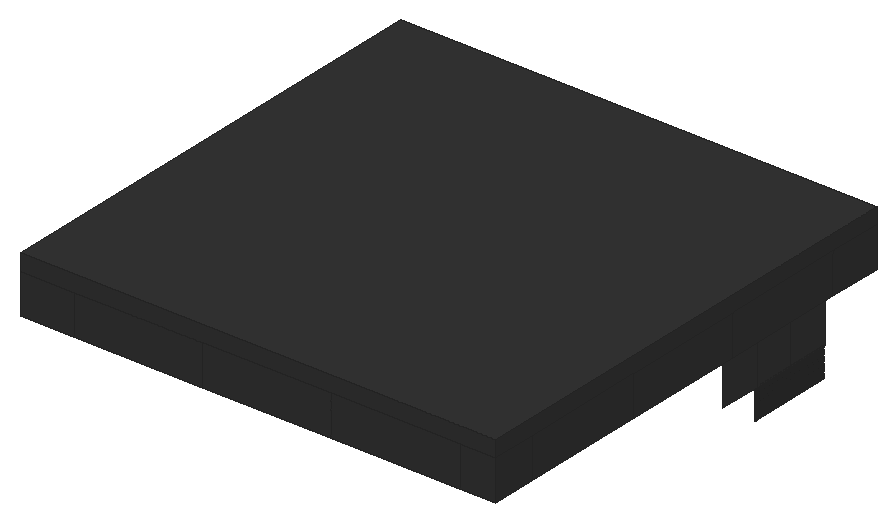
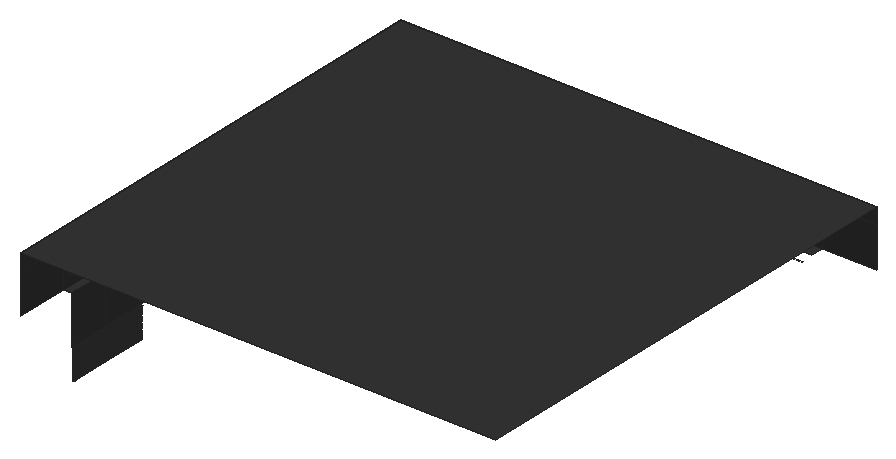
# SketchUp Ruby script. Lengths in inches.
U = 1.inch
M = Sketchup.active_model
def pt(a) = Geom::Point3d.new(a.map { |v| v * U })
def face(e, loops, mat)
  f = e.add_face(loops[0].map { |a| pt(a) })
  loops[1..].each { |l| e.add_face(l.map { |a| pt(a) }).erase! }
  f.material = f.back_material = mat if mat
  f
end
# faces: each face lists its corners as indices into pts; further lists are holes
def faces(e, pts, list, mat = nil) = list.each { |f| face(e, (f[0].is_a?(Array) ? f : [f]).map { |l| l.map { |i| pts[i] } }, mat) }
# xy, xz, yz: faces in a plane at the given z, y or x. An outline is a flat list of corners, or four numbers for a rectangle; further outlines are holes
def ring(l) = l.size == 4 ? [[l[0], l[1]], [l[2], l[1]], [l[2], l[3]], [l[0], l[3]]] : l.each_slice(2).to_a
def flat(e, list, mat, &to3) = list.each { |f| face(e, (f[0].is_a?(Array) ? f : [f]).map { |l| ring(l).map { |u, v| to3.(u, v) } }, mat) }
def xy(e, z, list, mat = nil) = flat(e, list, mat) { |x, y| [x, y, z] }
def xz(e, y, list, mat = nil) = flat(e, list, mat) { |x, z| [x, y, z] }
def yz(e, x, list, mat = nil) = flat(e, list, mat) { |y, z| [x, y, z] }
def lines(e, pts, list) = list.each { |a, b| e.add_line(pt(pts[a]), pt(pts[b])) }
# prism: a flat outline (further loops are holes) pulled along v
def prism(e, loops, v, mat = nil)
  f = face(e, loops, mat); d = Geom::Vector3d.new(v.map { |x| x * U })
  f.pushpull(f.normal.samedirection?(d) ? d.length : -d.length)
end
def box(e, o, s, mat = nil) = prism(e, [[o, [o[0] + s[0], o[1], o[2]], [o[0] + s[0], o[1] + s[1], o[2]], [o[0], o[1] + s[1], o[2]]]], [0, 0, s[2]], mat)
def at(x, y, z, deg = 0) = Geom::Transformation.translation(pt([x, y, z])) * Geom::Transformation.rotation(ORIGIN, Z_AXIS, deg.degrees)
def axes(o, x, y, z) = Geom::Transformation.new([*x, 0, *y, 0, *z, 0, *pt(o).to_a, 1])
def part(name) = M.definitions.add(name)
# library, detail: a bought-in or finely detailed component or shape, given as its bounding box
def library(name, o, s) = part(name).tap { |d| box(d.entities, o, s) }
def detail(e, o, s) = box(e.add_group.entities, o, s)
def put(e, d, t, mat = nil) = e.add_instance(d, t).tap { |i| i.material = mat if mat }
def group(e, t, mat = nil) = e.add_group.tap { |g| g.transformation = t; g.material = mat if mat }.entities
root = M.entities
M.materials.add("[0135_DarkGray]").color = [51, 51, 51]
M.materials.add("[0135_DarkGray]1").color = [53, 53, 53]
xy(root,480.06,[[1035.97,1165.35,1036.3125,1278.6875]],"[0135_DarkGray]1")
xy(root,482.66,[[1035.96,1165.35,1036.3,1278.6875]],"[0135_DarkGray]1")
xy(root,484.19,[[1035.97,1165.35,1036.3125,1278.6875]],"[0135_DarkGray]1")
xy(root,490.93,[[1035.96,1165.35,1036.3,1278.6875]],"[0135_DarkGray]1")
xy(root,492.46,[[1035.97,1165.35,1036.3125,1278.6875]],"[0135_DarkGray]1")
xy(root,496.59,[[1035.97,1165.35,1036.3125,1278.6875]],"[0135_DarkGray]1")
xy(root,503.33,[[1035.96,1165.35,1036.3,1278.6875]],"[0135_DarkGray]1")
xy(root,504.86,[[1035.97,1165.35,1036.3125,1278.6875]],"[0135_DarkGray]1")
xy(root,507.46,[[1035.96,1165.35,1036.3,1278.6875]],"[0135_DarkGray]1")
xy(root,508.99,[[1035.97,1165.35,1036.3125,1278.6875]],"[0135_DarkGray]1")
xy(root,513.125,[[1035.97,1165.35,1036.3125,1278.6875]],"[0135_DarkGray]1")
xy(root,515.73,[[1035.96,1165.35,1036.3,1278.6875]],"[0135_DarkGray]1")
xy(root,517.26,[[1035.97,1165.35,1036.3125,1278.6875]],"[0135_DarkGray]1")
xy(root,519.86,[[1035.96,1165.35,1036.3,1278.6875]],"[0135_DarkGray]1")
xy(root,520.4375,[[1034.13,1165.35,1038.13,1222.02],[1034.13,1222.02,1038.13,1278.6875]],"[0135_DarkGray]1")
xy(root,572.5,[[497.69,732.5625,579.69,734.5625],[585.69,732.5625,661.69,737.5625],[667.69,732.5625,743.69,737.5625],[749.69,732.5625,825.69,737.5625],[831.69,732.5625,907.69,737.5625],
  [913.69,732.5625,989.69,737.5625],[1028.13,774.6875,1033.13,856.6875],[1028.13,862.6875,1033.13,938.6875],[1028.13,944.6875,1033.13,1020.6875],[1028.13,1026.6875,1033.13,1102.6875]],"[0135_DarkGray]1")
xy(root,584.5,[[485.69,714.6875,485.69,732.5625,1001.69,732.5625,1001.69,727.5625,1038.13,727.5625,1038.13,762.6875,1033.13,762.6875,1033.13,1108.6875,1038.13,1108.6875,1038.13,1278.6875,1049.69,1278.6875,1049.69,714.6875]],"[0135_DarkGray]1")
xy(root,660,[[413.69,714.6875,1049.69,1350.6875]],"[0135_DarkGray]1")
xz(root,714.6875,[[413.69,584.5,485.69,638.14],[485.69,584.5,657.63,638.14],[657.63,584.5,829.57,638.14],[829.57,584.5,1001.51,638.14],[1001.51,584.5,1049.69,638.14],
  [413.69,638.14,1049.69,660]],"[0135_DarkGray]")
yz(root,1034.83,[[1165.35,481.18,1278.6875,481.52],[1165.35,485.3125,1278.6875,485.66],[1165.35,489.45,1278.6875,489.79],[1165.35,493.58,1278.6875,493.92],[1165.35,497.71,1278.6875,498.06],
  [1165.35,501.85,1278.6875,502.19],[1165.35,505.98,1278.6875,506.32],[1165.35,510.11,1278.6875,510.46],[1165.35,514.25,1278.6875,514.59],[1165.35,518.38,1278.6875,518.72]],"[0135_DarkGray]1")
yz(root,1038.13,[[1108.6875,520.4375,1165.35,584.5],[1165.35,520.4375,1222.02,584.5],[1222.02,520.4375,1278.6875,584.5]],"[0135_DarkGray]1")
yz(root,1049.69,[[714.6875,584.5,775.8125,638.14],[775.8125,584.5,943.4375,638.14],[943.4375,584.5,1111.0625,638.14],[1111.0625,584.5,1278.6875,638.14],[1278.6875,584.5,1350.6875,638.14],
  [714.6875,638.14,1350.6875,660]],"[0135_DarkGray]")
p = [[1035.64,1165.35,480.14],[1035.34,1165.35,480.3125],[1035.34,1278.6875,480.3125],[1035.64,1278.6875,480.14],[1035.97,1165.35,480.06],[1035.97,1278.6875,480.06],
  [1036.64,1165.35,480.15],[1036.3125,1165.35,480.06],[1036.3125,1278.6875,480.06],[1036.64,1278.6875,480.15],[1036.94,1165.35,480.32],[1036.94,1278.6875,480.32],
  [1035.1,1165.35,480.55],[1035.1,1278.6875,480.55],[1037.18,1165.35,480.57],[1037.18,1278.6875,480.57],[1034.93,1165.35,480.85],[1034.93,1278.6875,480.85],
  [1037.35,1165.35,480.86],[1037.35,1278.6875,480.86],[1034.83,1165.35,481.18],[1034.83,1278.6875,481.18],[1037.4375,1165.35,481.2],[1037.4375,1278.6875,481.2],
  [1037.44,1165.35,481.54],[1037.44,1278.6875,481.54],[1034.83,1165.35,481.52],[1034.92,1165.35,481.85],[1034.92,1278.6875,481.85],[1034.83,1278.6875,481.52],
  [1037.34,1165.35,481.87],[1037.34,1278.6875,481.87],[1035.09,1165.35,482.15],[1035.09,1278.6875,482.15],[1037.17,1165.35,482.16],[1037.17,1278.6875,482.16],
  [1035.33,1165.35,482.4],[1035.33,1278.6875,482.4],[1036.93,1165.35,482.41],[1036.93,1278.6875,482.41],[1035.625,1165.35,482.57],[1035.625,1278.6875,482.57],
  [1036.63,1165.35,482.57],[1036.63,1278.6875,482.57],[1035.96,1165.35,482.66],[1035.96,1278.6875,482.66],[1036.3,1165.35,482.66],[1036.3,1278.6875,482.66],
  [1035.97,1165.35,484.19],[1035.64,1165.35,484.28],[1035.64,1278.6875,484.28],[1035.97,1278.6875,484.19],[1036.64,1165.35,484.28],[1036.3125,1165.35,484.19],
  [1036.3125,1278.6875,484.19],[1036.64,1278.6875,484.28],[1035.34,1165.35,484.45],[1035.34,1278.6875,484.45],[1036.94,1165.35,484.46],[1036.94,1278.6875,484.46],
  [1035.1,1165.35,484.6875],[1035.1,1278.6875,484.6875],[1037.18,1165.35,484.7],[1037.18,1278.6875,484.7],[1034.93,1165.35,484.98],[1034.93,1278.6875,484.98],
  [1037.35,1165.35,485],[1037.35,1278.6875,485],[1034.83,1165.35,485.3125],[1034.83,1278.6875,485.3125],[1037.4375,1165.35,485.33],[1037.4375,1278.6875,485.33],
  [1037.44,1165.35,485.67],[1037.44,1278.6875,485.67],[1034.83,1165.35,485.66],[1034.92,1165.35,485.99],[1034.92,1278.6875,485.99],[1034.83,1278.6875,485.66],
  [1037.34,1165.35,486],[1037.34,1278.6875,486],[1035.09,1165.35,486.29],[1035.09,1278.6875,486.29],[1037.17,1165.35,486.3],[1037.17,1278.6875,486.3],
  [1035.33,1165.35,486.53],[1035.33,1278.6875,486.53],[1036.93,1165.35,486.54],[1036.93,1278.6875,486.54],[1035.625,1165.35,486.7],[1035.625,1278.6875,486.7],
  [1036.63,1165.35,486.71],[1036.63,1278.6875,486.71],[1035.96,1165.35,486.79],[1035.96,1278.6875,486.79],[1036.3,1165.35,486.8],[1036.3,1278.6875,486.8],
  [1035.97,1165.35,488.32],[1035.64,1165.35,488.41],[1035.64,1278.6875,488.41],[1035.97,1278.6875,488.32],[1036.3125,1165.35,488.33],[1036.3125,1278.6875,488.33],
  [1036.64,1165.35,488.42],[1036.64,1278.6875,488.42],[1035.34,1165.35,488.58],[1035.34,1278.6875,488.58],[1036.94,1165.35,488.59],[1036.94,1278.6875,488.59],
  [1035.1,1165.35,488.82],[1035.1,1278.6875,488.82],[1037.18,1165.35,488.83],[1037.18,1278.6875,488.83],[1034.93,1165.35,489.12],[1034.93,1278.6875,489.12],
  [1037.35,1165.35,489.13],[1037.35,1278.6875,489.13],[1034.83,1165.35,489.45],[1034.83,1278.6875,489.45],[1037.4375,1165.35,489.46],[1037.4375,1278.6875,489.46],
  [1037.44,1165.35,489.8],[1037.44,1278.6875,489.8],[1034.83,1165.35,489.79],[1034.92,1165.35,490.12],[1034.92,1278.6875,490.12],[1034.83,1278.6875,489.79],
  [1037.34,1165.35,490.14],[1037.34,1278.6875,490.14],[1035.09,1165.35,490.42],[1035.09,1278.6875,490.42],[1037.17,1165.35,490.43],[1037.17,1278.6875,490.43],
  [1035.33,1165.35,490.66],[1035.33,1278.6875,490.66],[1036.93,1165.35,490.67],[1036.93,1278.6875,490.67],[1035.625,1165.35,490.84],[1035.625,1278.6875,490.84],
  [1036.63,1165.35,490.84],[1036.63,1278.6875,490.84],[1035.96,1165.35,490.93],[1035.96,1278.6875,490.93],[1036.3,1165.35,490.93],[1036.3,1278.6875,490.93],
  [1035.64,1165.35,492.54],[1035.34,1165.35,492.71],[1035.34,1278.6875,492.71],[1035.64,1278.6875,492.54],[1035.97,1165.35,492.46],[1035.97,1278.6875,492.46],
  [1036.64,1165.35,492.55],[1036.3125,1165.35,492.46],[1036.3125,1278.6875,492.46],[1036.64,1278.6875,492.55],[1036.94,1165.35,492.72],[1036.94,1278.6875,492.72],
  [1035.1,1165.35,492.95],[1035.1,1278.6875,492.95],[1037.18,1165.35,492.97],[1037.18,1278.6875,492.97],[1034.93,1165.35,493.25],[1034.93,1278.6875,493.25],
  [1037.35,1165.35,493.26],[1037.35,1278.6875,493.26],[1034.83,1165.35,493.58],[1034.83,1278.6875,493.58],[1037.4375,1165.35,493.6],[1037.4375,1278.6875,493.6],
  [1037.44,1165.35,493.9375],[1037.44,1278.6875,493.9375],[1034.83,1165.35,493.92],[1034.92,1165.35,494.25],[1034.92,1278.6875,494.25],[1034.83,1278.6875,493.92],
  [1037.34,1165.35,494.27],[1037.34,1278.6875,494.27],[1035.09,1165.35,494.55],[1035.09,1278.6875,494.55],[1037.17,1165.35,494.5625],[1037.17,1278.6875,494.5625],
  [1035.33,1165.35,494.8],[1035.33,1278.6875,494.8],[1036.93,1165.35,494.81],[1036.93,1278.6875,494.81],[1035.625,1165.35,494.97],[1035.625,1278.6875,494.97],
  [1036.63,1165.35,494.97],[1036.63,1278.6875,494.97],[1035.96,1165.35,495.06],[1035.96,1278.6875,495.06],[1036.3,1165.35,495.0625],[1036.3,1278.6875,495.0625],
  [1035.97,1165.35,496.59],[1035.64,1165.35,496.68],[1035.64,1278.6875,496.68],[1035.97,1278.6875,496.59],[1036.64,1165.35,496.68],[1036.3125,1165.35,496.59],
  [1036.3125,1278.6875,496.59],[1036.64,1278.6875,496.68],[1035.34,1165.35,496.85],[1035.34,1278.6875,496.85],[1036.94,1165.35,496.86],[1036.94,1278.6875,496.86],
  [1035.1,1165.35,497.09],[1035.1,1278.6875,497.09],[1037.18,1165.35,497.1],[1037.18,1278.6875,497.1],[1034.93,1165.35,497.38],[1034.93,1278.6875,497.38],
  [1037.35,1165.35,497.4],[1037.35,1278.6875,497.4],[1034.83,1165.35,497.71],[1034.83,1278.6875,497.71],[1037.4375,1165.35,497.73],[1037.4375,1278.6875,497.73],
  [1037.44,1165.35,498.07],[1037.44,1278.6875,498.07],[1034.83,1165.35,498.06],[1034.92,1165.35,498.39],[1034.92,1278.6875,498.39],[1034.83,1278.6875,498.06],
  [1037.34,1165.35,498.4],[1037.34,1278.6875,498.4],[1035.09,1165.35,498.6875],[1035.09,1278.6875,498.6875],[1037.17,1165.35,498.7],[1037.17,1278.6875,498.7],
  [1035.33,1165.35,498.93],[1035.33,1278.6875,498.93],[1036.93,1165.35,498.9375],[1036.93,1278.6875,498.9375],[1035.625,1165.35,499.1],[1035.625,1278.6875,499.1],
  [1036.63,1165.35,499.11],[1036.63,1278.6875,499.11],[1035.96,1165.35,499.19],[1035.96,1278.6875,499.19],[1036.3,1165.35,499.2],[1036.3,1278.6875,499.2],
  [1035.97,1165.35,500.72],[1035.64,1165.35,500.8125],[1035.64,1278.6875,500.8125],[1035.97,1278.6875,500.72],[1036.3125,1165.35,500.73],[1036.3125,1278.6875,500.73],
  [1036.64,1165.35,500.82],[1036.64,1278.6875,500.82],[1035.34,1165.35,500.98],[1035.34,1278.6875,500.98],[1036.94,1165.35,500.99],[1036.94,1278.6875,500.99],
  [1035.1,1165.35,501.22],[1035.1,1278.6875,501.22],[1037.18,1165.35,501.23],[1037.18,1278.6875,501.23],[1034.93,1165.35,501.52],[1034.93,1278.6875,501.52],
  [1037.35,1165.35,501.53],[1037.35,1278.6875,501.53],[1034.83,1165.35,501.85],[1034.83,1278.6875,501.85],[1037.4375,1165.35,501.86],[1037.4375,1278.6875,501.86],
  [1037.44,1165.35,502.2],[1037.44,1278.6875,502.2],[1034.83,1165.35,502.19],[1034.92,1165.35,502.52],[1034.92,1278.6875,502.52],[1034.83,1278.6875,502.19],
  [1037.34,1165.35,502.54],[1037.34,1278.6875,502.54],[1035.09,1165.35,502.82],[1035.09,1278.6875,502.82],[1037.17,1165.35,502.83],[1037.17,1278.6875,502.83],
  [1035.33,1165.35,503.0625],[1035.33,1278.6875,503.0625],[1036.93,1165.35,503.07],[1036.93,1278.6875,503.07],[1035.625,1165.35,503.24],[1035.625,1278.6875,503.24],
  [1036.63,1165.35,503.24],[1036.63,1278.6875,503.24],[1035.96,1165.35,503.33],[1035.96,1278.6875,503.33],[1036.3,1165.35,503.33],[1036.3,1278.6875,503.33],
  [1035.64,1165.35,504.94],[1035.34,1165.35,505.11],[1035.34,1278.6875,505.11],[1035.64,1278.6875,504.94],[1035.97,1165.35,504.86],[1035.97,1278.6875,504.86],
  [1036.64,1165.35,504.95],[1036.3125,1165.35,504.86],[1036.3125,1278.6875,504.86],[1036.64,1278.6875,504.95],[1036.94,1165.35,505.12],[1036.94,1278.6875,505.12],
  [1035.1,1165.35,505.35],[1035.1,1278.6875,505.35],[1037.18,1165.35,505.37],[1037.18,1278.6875,505.37],[1034.93,1165.35,505.65],[1034.93,1278.6875,505.65],
  [1037.35,1165.35,505.66],[1037.35,1278.6875,505.66],[1034.83,1165.35,505.98],[1034.83,1278.6875,505.98],[1037.4375,1165.35,506],[1037.4375,1278.6875,506],
  [1037.44,1165.35,506.34],[1037.44,1278.6875,506.34],[1034.83,1165.35,506.32],[1034.92,1165.35,506.65],[1034.92,1278.6875,506.65],[1034.83,1278.6875,506.32],
  [1037.34,1165.35,506.67],[1037.34,1278.6875,506.67],[1035.09,1165.35,506.95],[1035.09,1278.6875,506.95],[1037.17,1165.35,506.96],[1037.17,1278.6875,506.96],
  [1035.33,1165.35,507.2],[1035.33,1278.6875,507.2],[1036.93,1165.35,507.21],[1036.93,1278.6875,507.21],[1035.625,1165.35,507.37],[1035.625,1278.6875,507.37],
  [1036.63,1165.35,507.375],[1036.63,1278.6875,507.375],[1035.96,1165.35,507.46],[1035.96,1278.6875,507.46],[1036.3,1165.35,507.46],[1036.3,1278.6875,507.46],
  [1035.97,1165.35,508.99],[1035.64,1165.35,509.08],[1035.64,1278.6875,509.08],[1035.97,1278.6875,508.99],[1036.64,1165.35,509.08],[1036.3125,1165.35,508.99],
  [1036.3125,1278.6875,508.99],[1036.64,1278.6875,509.08],[1035.34,1165.35,509.25],[1035.34,1278.6875,509.25],[1036.94,1165.35,509.26],[1036.94,1278.6875,509.26],
  [1035.1,1165.35,509.49],[1035.1,1278.6875,509.49],[1037.18,1165.35,509.5],[1037.18,1278.6875,509.5],[1034.93,1165.35,509.78],[1034.93,1278.6875,509.78],
  [1037.35,1165.35,509.8],[1037.35,1278.6875,509.8],[1034.83,1165.35,510.11],[1034.83,1278.6875,510.11],[1037.4375,1165.35,510.13],[1037.4375,1278.6875,510.13],
  [1037.44,1165.35,510.47],[1037.44,1278.6875,510.47],[1034.83,1165.35,510.46],[1034.92,1165.35,510.79],[1034.92,1278.6875,510.79],[1034.83,1278.6875,510.46],
  [1037.34,1165.35,510.8],[1037.34,1278.6875,510.8],[1035.09,1165.35,511.09],[1035.09,1278.6875,511.09],[1037.17,1165.35,511.1],[1037.17,1278.6875,511.1],
  [1035.33,1165.35,511.33],[1035.33,1278.6875,511.33],[1036.93,1165.35,511.34],[1036.93,1278.6875,511.34],[1035.625,1165.35,511.5],[1035.625,1278.6875,511.5],
  [1036.63,1165.35,511.51],[1036.63,1278.6875,511.51],[1035.96,1165.35,511.59],[1035.96,1278.6875,511.59],[1036.3,1165.35,511.6],[1036.3,1278.6875,511.6],
  [1035.97,1165.35,513.125],[1035.64,1165.35,513.21],[1035.64,1278.6875,513.21],[1035.97,1278.6875,513.125],[1036.64,1165.35,513.22],[1036.3125,1165.35,513.125],
  [1036.3125,1278.6875,513.125],[1036.64,1278.6875,513.22],[1035.34,1165.35,513.38],[1035.34,1278.6875,513.38],[1036.94,1165.35,513.39],[1036.94,1278.6875,513.39],
  [1035.1,1165.35,513.62],[1035.1,1278.6875,513.62],[1037.18,1165.35,513.63],[1037.18,1278.6875,513.63],[1034.93,1165.35,513.92],[1034.93,1278.6875,513.92],
  [1037.35,1165.35,513.93],[1037.35,1278.6875,513.93],[1034.83,1165.35,514.25],[1034.83,1278.6875,514.25],[1037.4375,1165.35,514.26],[1037.4375,1278.6875,514.26],
  [1037.44,1165.35,514.6],[1037.44,1278.6875,514.6],[1034.83,1165.35,514.59],[1034.92,1165.35,514.92],[1034.92,1278.6875,514.92],[1034.83,1278.6875,514.59],
  [1037.34,1165.35,514.94],[1037.34,1278.6875,514.94],[1035.09,1165.35,515.22],[1035.09,1278.6875,515.22],[1037.17,1165.35,515.23],[1037.17,1278.6875,515.23],
  [1035.33,1165.35,515.46],[1035.33,1278.6875,515.46],[1036.93,1165.35,515.47],[1036.93,1278.6875,515.47],[1035.625,1165.35,515.64],[1035.625,1278.6875,515.64],
  [1036.63,1165.35,515.64],[1036.63,1278.6875,515.64],[1035.96,1165.35,515.73],[1035.96,1278.6875,515.73],[1036.3,1165.35,515.73],[1036.3,1278.6875,515.73],
  [1035.64,1165.35,517.34],[1035.34,1165.35,517.51],[1035.34,1278.6875,517.51],[1035.64,1278.6875,517.34],[1035.97,1165.35,517.26],[1035.97,1278.6875,517.26],
  [1036.64,1165.35,517.35],[1036.3125,1165.35,517.26],[1036.3125,1278.6875,517.26],[1036.64,1278.6875,517.35],[1036.94,1165.35,517.52],[1036.94,1278.6875,517.52],
  [1035.1,1165.35,517.75],[1035.1,1278.6875,517.75],[1037.18,1165.35,517.77],[1037.18,1278.6875,517.77],[1034.93,1165.35,518.05],[1034.93,1278.6875,518.05],
  [1037.35,1165.35,518.0625],[1037.35,1278.6875,518.0625],[1034.83,1165.35,518.38],[1034.83,1278.6875,518.38],[1037.4375,1165.35,518.4],[1037.4375,1278.6875,518.4],
  [1037.44,1165.35,518.74],[1037.44,1278.6875,518.74],[1034.83,1165.35,518.72],[1034.92,1165.35,519.05],[1034.92,1278.6875,519.05],[1034.83,1278.6875,518.72],
  [1037.34,1165.35,519.07],[1037.34,1278.6875,519.07],[1035.09,1165.35,519.35],[1035.09,1278.6875,519.35],[1037.17,1165.35,519.36],[1037.17,1278.6875,519.36],
  [1035.33,1165.35,519.6],[1035.33,1278.6875,519.6],[1036.93,1165.35,519.61],[1036.93,1278.6875,519.61],[1035.625,1165.35,519.77],[1035.625,1278.6875,519.77],
  [1036.63,1165.35,519.77],[1036.63,1278.6875,519.77],[1035.96,1165.35,519.86],[1035.96,1278.6875,519.86],[1036.3,1165.35,519.86],[1036.3,1278.6875,519.86]]
faces(root,p,[[0,1,2,3],[4,0,3,5],[6,7,8,9],[10,6,9,11],[1,12,13,2],[14,10,11,15],[12,16,17,13],[18,14,15,19],
  [16,20,21,17],[22,18,19,23],[24,22,23,25],[26,27,28,29],[30,24,25,31],[27,32,33,28],[34,30,31,35],[32,36,37,33],
  [38,34,35,39],[36,40,41,37],[42,38,39,43],[40,44,45,41],[46,42,43,47],[48,49,50,51],[52,53,54,55],[49,56,57,50],
  [58,52,55,59],[56,60,61,57],[62,58,59,63],[60,64,65,61],[66,62,63,67],[64,68,69,65],[70,66,67,71],[72,70,71,73],
  [74,75,76,77],[78,72,73,79],[75,80,81,76],[82,78,79,83],[80,84,85,81],[86,82,83,87],[84,88,89,85],[90,86,87,91],
  [88,92,93,89],[94,90,91,95],[92,94,95,93],[96,97,98,99],[100,96,99,101],[102,100,101,103],[97,104,105,98],[106,102,103,107],
  [104,108,109,105],[110,106,107,111],[108,112,113,109],[114,110,111,115],[112,116,117,113],[118,114,115,119],[120,118,119,121],[122,123,124,125],
  [126,120,121,127],[123,128,129,124],[130,126,127,131],[128,132,133,129],[134,130,131,135],[132,136,137,133],[138,134,135,139],[136,140,141,137],
  [142,138,139,143],[144,145,146,147],[148,144,147,149],[150,151,152,153],[154,150,153,155],[145,156,157,146],[158,154,155,159],[156,160,161,157],
  [162,158,159,163],[160,164,165,161],[166,162,163,167],[168,166,167,169],[170,171,172,173],[174,168,169,175],[171,176,177,172],[178,174,175,179],
  [176,180,181,177],[182,178,179,183],[180,184,185,181],[186,182,183,187],[184,188,189,185],[190,186,187,191],[188,190,191,189],[192,193,194,195],
  [196,197,198,199],[193,200,201,194],[202,196,199,203],[200,204,205,201],[206,202,203,207],[204,208,209,205],[210,206,207,211],[208,212,213,209],
  [214,210,211,215],[216,214,215,217],[218,219,220,221],[222,216,217,223],[219,224,225,220],[226,222,223,227],[224,228,229,225],[230,226,227,231],
  [228,232,233,229],[234,230,231,235],[232,236,237,233],[238,234,235,239],[236,238,239,237],[240,241,242,243],[244,240,243,245],[246,244,245,247],
  [241,248,249,242],[250,246,247,251],[248,252,253,249],[254,250,251,255],[252,256,257,253],[258,254,255,259],[256,260,261,257],[262,258,259,263],
  [264,262,263,265],[266,267,268,269],[270,264,265,271],[267,272,273,268],[274,270,271,275],[272,276,277,273],[278,274,275,279],[276,280,281,277],
  [282,278,279,283],[280,284,285,281],[286,282,283,287],[288,289,290,291],[292,288,291,293],[294,295,296,297],[298,294,297,299],[289,300,301,290],
  [302,298,299,303],[300,304,305,301],[306,302,303,307],[304,308,309,305],[310,306,307,311],[312,310,311,313],[314,315,316,317],[318,312,313,319],
  [315,320,321,316],[322,318,319,323],[320,324,325,321],[326,322,323,327],[324,328,329,325],[330,326,327,331],[328,332,333,329],[334,330,331,335],
  [336,337,338,339],[340,341,342,343],[337,344,345,338],[346,340,343,347],[344,348,349,345],[350,346,347,351],[348,352,353,349],[354,350,351,355],
  [352,356,357,353],[358,354,355,359],[360,358,359,361],[362,363,364,365],[366,360,361,367],[363,368,369,364],[370,366,367,371],[368,372,373,369],
  [374,370,371,375],[372,376,377,373],[378,374,375,379],[376,380,381,377],[382,378,379,383],[380,382,383,381],[384,385,386,387],[388,389,390,391],
  [385,392,393,386],[394,388,391,395],[392,396,397,393],[398,394,395,399],[396,400,401,397],[402,398,399,403],[400,404,405,401],[406,402,403,407],
  [408,406,407,409],[410,411,412,413],[414,408,409,415],[411,416,417,412],[418,414,415,419],[416,420,421,417],[422,418,419,423],[420,424,425,421],
  [426,422,423,427],[424,428,429,425],[430,426,427,431],[432,433,434,435],[436,432,435,437],[438,439,440,441],[442,438,441,443],[433,444,445,434],
  [446,442,443,447],[444,448,449,445],[450,446,447,451],[448,452,453,449],[454,450,451,455],[456,454,455,457],[458,459,460,461],[462,456,457,463],
  [459,464,465,460],[466,462,463,467],[464,468,469,465],[470,466,467,471],[468,472,473,469],[474,470,471,475],[472,476,477,473],[478,474,475,479]],"[0135_DarkGray]1")
